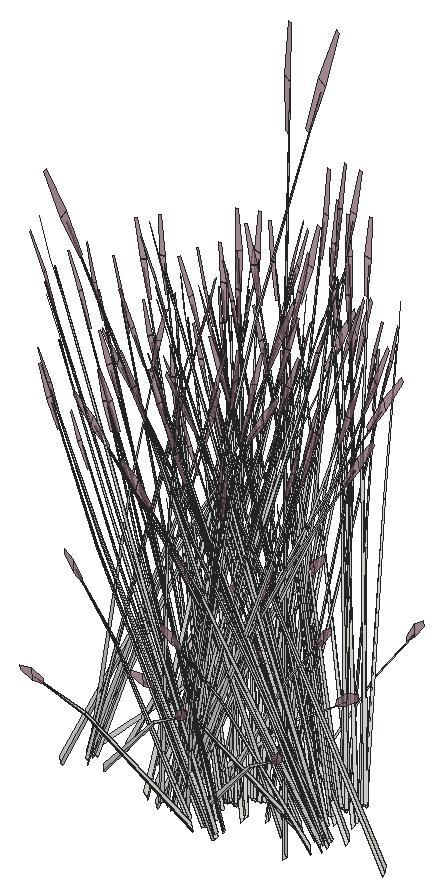
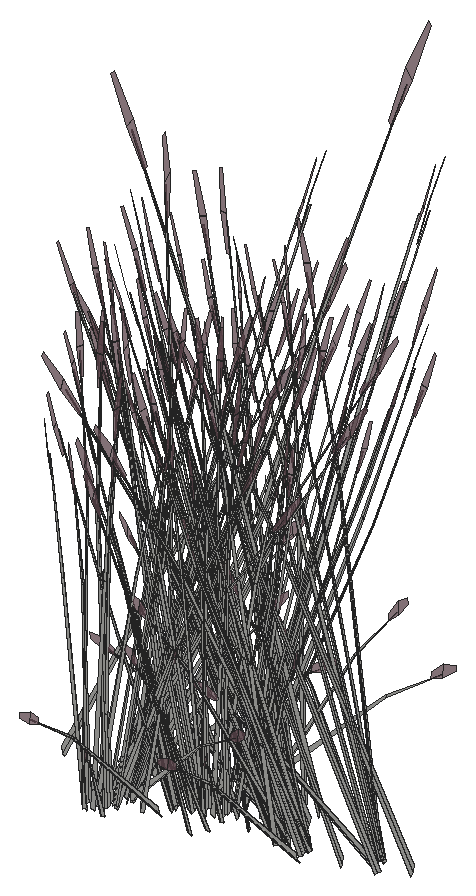
# SketchUp Ruby script. Lengths in inches.
U = 1.inch
M = Sketchup.active_model
def pt(a) = Geom::Point3d.new(a.map { |v| v * U })
def face(e, loops, mat)
  f = e.add_face(loops[0].map { |a| pt(a) })
  loops[1..].each { |l| e.add_face(l.map { |a| pt(a) }).erase! }
  f.material = f.back_material = mat if mat
  f
end
# faces: each face lists its corners as indices into pts; further lists are holes
def faces(e, pts, list, mat = nil) = list.each { |f| face(e, (f[0].is_a?(Array) ? f : [f]).map { |l| l.map { |i| pts[i] } }, mat) }
# xy, xz, yz: faces in a plane at the given z, y or x. An outline is a flat list of corners, or four numbers for a rectangle; further outlines are holes
def ring(l) = l.size == 4 ? [[l[0], l[1]], [l[2], l[1]], [l[2], l[3]], [l[0], l[3]]] : l.each_slice(2).to_a
def flat(e, list, mat, &to3) = list.each { |f| face(e, (f[0].is_a?(Array) ? f : [f]).map { |l| ring(l).map { |u, v| to3.(u, v) } }, mat) }
def xy(e, z, list, mat = nil) = flat(e, list, mat) { |x, y| [x, y, z] }
def xz(e, y, list, mat = nil) = flat(e, list, mat) { |x, z| [x, y, z] }
def yz(e, x, list, mat = nil) = flat(e, list, mat) { |y, z| [x, y, z] }
def lines(e, pts, list) = list.each { |a, b| e.add_line(pt(pts[a]), pt(pts[b])) }
# prism: a flat outline (further loops are holes) pulled along v
def prism(e, loops, v, mat = nil)
  f = face(e, loops, mat); d = Geom::Vector3d.new(v.map { |x| x * U })
  f.pushpull(f.normal.samedirection?(d) ? d.length : -d.length)
end
def box(e, o, s, mat = nil) = prism(e, [[o, [o[0] + s[0], o[1], o[2]], [o[0] + s[0], o[1] + s[1], o[2]], [o[0], o[1] + s[1], o[2]]]], [0, 0, s[2]], mat)
def at(x, y, z, deg = 0) = Geom::Transformation.translation(pt([x, y, z])) * Geom::Transformation.rotation(ORIGIN, Z_AXIS, deg.degrees)
def axes(o, x, y, z) = Geom::Transformation.new([*x, 0, *y, 0, *z, 0, *pt(o).to_a, 1])
def part(name) = M.definitions.add(name)
# library, detail: a bought-in or finely detailed component or shape, given as its bounding box
def library(name, o, s) = part(name).tap { |d| box(d.entities, o, s) }
def detail(e, o, s) = box(e.add_group.entities, o, s)
def put(e, d, t, mat = nil) = e.add_instance(d, t).tap { |i| i.material = mat if mat }
def group(e, t, mat = nil) = e.add_group.tap { |g| g.transformation = t; g.material = mat if mat }.entities
root = M.entities
M.materials.add("LightPink_Translucent").color = [144, 107, 117]
M.materials["LightPink_Translucent"].alpha = 0.75
c1 = part("blade")
p = [[2.15,0.21,22],[0,0.17,0],[0.09,0.45,0],[2.18,0.31,22],[2.29,0.31,22],[0.38,0.45,0],
  [2.48,0.24,33],[2.49,0.24,33],[2.48,0.22,33]]
faces(c1.entities,p,[[0,1,2,3],[4,5,2,3],[6,3,4,7],[8,0,3,6]])
c2 = part("seeds")
p = [[0.3,-0.1,1.38],[-0.01,-0.03,1.59],[-0.01,-0.03,0.03],[0.14,-0.07,-0.07],[0.29,-0.03,3],[0.15,0.01,3.11]]
faces(c2.entities,p,[[0,1,2,3],[1,0,4,5]],"LightPink_Translucent")
c3 = part("blade with seeds")
put(c3.entities,c1,at(0,0,0))
put(c3.entities,c2,axes([2.4,0.25,30.99],[1.5799,-0.05474,1.17369],[-0.12525,1.92788,0.29478],[-0.07173,-0.02425,1.56792]))
put(root,c3,axes([663.24,337.52,268.18],[-0.32734,-0.51701,-0.10093],[0.58097,-0.25407,-0.56021],[0.24483,-0.06821,0.85122]))
put(root,c3,axes([663.46,337.375,267.93],[-0.18381,0.5206,0.39842],[-0.60429,-0.17802,0.32852],[0.23764,-0.03129,0.82444]))
put(root,c3,axes([670.3125,337.49,267.91],[0.08303,0.01531,1.47228],[0.25685,0.50448,-0.13912],[-0.16996,0.13241,0.26054]))
put(root,c3,axes([672.2,336.875,267.89],[-0.17625,0.51936,-0.42412],[-0.60429,-0.17802,-0.32852],[-0.2433,0.04762,0.81151]))
put(root,c3,axes([672.66,335.75,267.89],[-0.47241,0.37822,-0.42412],[-0.41372,-0.39954,-0.32852],[-0.24002,-0.05755,0.81151]))
put(root,c3,axes([666.25,339.77,267.91],[0.08247,0.09194,1.45204],[0.66552,0.03612,-0.22964],[0.06692,0.20277,0.11645]))
put(root,c3,axes([671.99,334.69,267.91],[0.04823,0.05698,1.47228],[-0.23252,0.51221,-0.13912],[-0.23548,0.00371,0.26054]))
put(root,c3,axes([663.08,338.25,267.91],[0.13956,-0.00966,1.45204],[0.38281,-0.44358,-0.22964],[0.24825,0.05855,0.11645]))
put(root,c3,axes([672.53,334.35,267.91],[-0.13998,-0.00403,1.45204],[-0.44565,0.40302,-0.22964],[-0.23779,-0.08235,0.11645]))
put(root,c3,axes([666.59,338.53,268.19],[0.19614,-0.43908,0.29394],[0.57222,0.12807,-0.37948],[0.05247,0.17678,0.72609]))
put(root,c3,axes([663.21,337.08,267.89],[0.17625,-0.51936,-0.42412],[0.60429,0.17802,-0.32852],[0.2433,-0.04762,0.81151]))
put(root,c3,axes([671.96,336.58,267.93],[0.18381,-0.5206,0.39842],[0.60429,0.17802,0.32852],[-0.23764,0.03129,0.82444]))
put(root,c3,axes([672.17,336.43,268.18],[0.32734,0.51701,-0.10093],[-0.58097,0.25407,-0.56021],[-0.24483,0.06821,0.85122]))
put(root,c3,axes([672.91,335.36,268.18],[-0.03484,0.58066,-0.10093],[-0.65957,-0.01587,-0.56021],[-0.25402,-0.04034,0.85122]))
put(root,c3,axes([672.49,335.4,267.76],[-0.37017,-0.35748,-0.29394],[0.42268,-0.3384,0.37948],[-0.21476,-0.05149,0.72609]))
put(root,c3,axes([671.91,336.44,267.93],[-0.23895,-0.38931,0.05337],[0.43573,-0.19055,0.42015],[-0.19208,0.0376,0.64067]))
put(root,c3,axes([673.01,337.52,267.22],[0.1625,-0.17544,1.42242],[0.41029,0.47354,0.11501],[-0.28141,0.21565,0.60807]))
put(root,c3,axes([672.03,337.98,267.76],[-0.56631,0.0816,-0.29394],[-0.14954,-0.46647,0.37948],[-0.16229,0.12529,0.72609]))
put(root,c3,axes([663.58,337.32,267.76],[0.54068,0.15928,-0.29394],[-0.1577,0.46469,0.37948],[0.21769,-0.04261,0.72609]))
put(root,c3,axes([666.71,338.6,268.13],[0.31051,0.46426,-0.58968],[-0.63919,0.25873,0.07116],[0.07261,0.22432,0.83415]))
put(root,c3,axes([662.54,338.32,268.13],[0.65035,0.01375,-0.58968],[-0.04368,0.5789,0.07116],[0.27552,0.06109,0.83415]))
put(root,c3,axes([667.36,340.1,268.6875],[0.44958,-0.32756,-0.05385],[0.41194,0.35875,-0.24415],[0.029,0.10165,0.8053]))
put(root,c3,axes([672.1,337.875,267.93],[-0.16135,-0.52549,0.39842],[0.63294,-0.0912,0.32852],[-0.18654,0.12359,0.82444]))
put(root,c3,axes([664.54,339.06,267.91],[-0.05883,-0.04999,1.47228],[0.12868,-0.53581,-0.13912],[0.23172,-0.03423,0.26054]))
put(root,c3,axes([662.11,336.74,267.22],[-0.26985,0.01293,1.42242],[0.17902,-0.56047,0.11501],[0.38456,0.03467,0.60807]))
put(root,c3,axes([672.43,335.26,268.23],[0.53728,-0.42137,0.44623],[0.46337,0.44748,0.36794],[-0.25207,-0.07773,0.92337]))
put(root,c3,axes([671.98,337.78,267.93],[-0.44663,-0.24013,0.05337],[0.26003,-0.34195,0.42015],[-0.14319,0.11055,0.64067]))
put(root,c3,axes([666.95,338.69,267.89],[0.63954,0.14313,-0.42412],[-0.21921,0.49074,-0.32852],[0.05864,0.19758,0.81151]))
put(root,c3,axes([666.4,338.72,268.18],[0.63664,-0.26583,-0.10093],[0.31286,0.47181,-0.56021],[0.084,0.19882,0.85122]))
put(root,c3,axes([663.1,337.27,268.13],[0.57168,-0.25217,-0.58968],[0.3186,0.51908,0.07116],[0.27622,-0.05897,0.83415]))
put(root,c3,axes([672.89,337.95,267.22],[0.12114,-0.19625,1.42242],[0.50818,0.40613,0.11501],[-0.22925,0.25313,0.60807]))
put(root,c3,axes([672.4,336.59,268.19],[0.54068,0.15928,0.29394],[-0.1577,0.46469,-0.37948],[-0.21769,0.04261,0.72609]))
put(root,c3,axes([665.02,336.71,267.91],[0.09028,-0.08697,1.45204],[-0.11555,-0.53348,-0.22964],[0.22652,-0.10115,0.11645]))
put(root,c3,axes([672.5,338.03,267.89],[0.16713,0.52135,-0.42412],[-0.63294,0.0912,-0.32852],[-0.18138,0.14003,0.81151]))
put(root,c3,axes([672.68,335.26,267.93],[0.03276,-0.43418,0.05337],[0.49468,0.0119,0.42015],[-0.18949,-0.04543,0.64067]))
put(root,c3,axes([671.51,338.97,267.91],[-0.01617,0.11299,1.45204],[0.45894,0.39307,-0.22964],[-0.12015,0.18588,0.11645]))
put(root,c3,axes([674.2,334.51,268.51],[-0.4342,0.54737,-0.11304],[-0.6288,-0.31535,-0.62743],[-0.21858,-0.15465,0.95337]))
put(root,c3,axes([673.01,335.58,268.19],[0.37017,0.35748,0.29394],[-0.42268,0.3384,-0.37948],[-0.21476,-0.05149,0.72609]))
put(root,c3,axes([673.75,334.97,267.89],[-0.64198,0.13573,-0.42412],[-0.1123,-0.514,-0.32852],[-0.17243,-0.1473,0.81151]))
put(root,c3,axes([672.2,337.66,268.18],[0.60181,0.31483,-0.10093],[-0.34671,0.45593,-0.56021],[-0.17003,0.15849,0.85122]))
put(root,c3,axes([668.18,338.77,267.93],[-0.64708,0.13103,0.39842],[-0.1123,-0.514,0.32852],[0.15218,0.15149,0.82444]))
put(root,c3,axes([668.06,338.875,267.93],[-0.29569,0.36271,0.05337],[-0.42107,-0.21117,0.42015],[0.13613,0.11629,0.64067]))
put(root,c3,axes([667.31,337.68,267.22],[-0.14872,-0.18332,1.42242],[0.6872,-0.15433,0.11501],[0.15531,0.28779,0.60807]))
put(root,c3,axes([676.87,339.23,267.22],[0.26985,-0.01293,1.42242],[-0.17902,0.56047,0.11501],[-0.38456,-0.03467,0.60807]))
put(root,c3,axes([671.21,339.03,268.6875],[0.5741,0.15241,-0.05385],[-0.1766,0.46909,-0.24415],[-0.0939,0.07122,0.8053]))
put(root,c3,axes([672.49,337.7,268.19],[0.56631,-0.0816,0.29394],[0.14954,0.46647,-0.37948],[-0.16229,0.12529,0.72609]))
put(root,c3,axes([667.96,338.46,268.19],[-0.10048,-0.4599,0.29394],[0.5744,-0.12144,-0.37948],[0.15428,0.13179,0.72609]))
put(root,c3,axes([673.03,338.94,267.93],[-0.46327,-0.38957,0.39842],[0.49199,-0.33598,0.32852],[-0.08546,0.18277,0.82444]))
put(root,c3,axes([676.98,340.21,267.22],[0.22574,-0.12077,1.42242],[0.19004,0.55807,0.11501],[-0.35439,0.12613,0.60807]))
put(root,c3,axes([668.35,335.8125,267.71],[-0.56218,-0.29666,1.14775],[0.59361,-0.46189,0.49522],[0.18138,0.27836,1.10941]))
put(root,c3,axes([667.4,339.1,267.91],[0.00193,-0.06913,1.47228],[0.55753,-0.30498,-0.13912],[0.19366,0.10886,0.26054]))
put(root,c3,axes([672.86,338.9,267.93],[-0.53464,-0.0266,0.05337],[0.01466,-0.40172,0.42015],[-0.05594,0.15388,0.64067]))
put(root,c3,axes([673.03,339.06,267.76],[-0.4402,0.30062,-0.29394],[-0.41671,-0.34326,0.37948],[-0.0634,0.1744,0.72609]))
put(root,c3,axes([678.28,339.63,266.77],[0.18493,-0.0826,1.46963],[0.06377,0.5767,0.11501],[-0.40056,0.07652,0.52526]))
put(root,c3,axes([674.16,334.96,268.19],[0.10048,0.4599,0.29394],[-0.5744,0.12144,-0.37948],[-0.15428,-0.13179,0.72609]))
put(root,c3,axes([671.46,340.125,267.91],[0.07381,-0.03447,1.47228],[0.61004,0.22929,-0.13912],[-0.01434,0.19091,0.26054]))
put(root,c3,axes([675.34,338.07,266.76],[0.56221,0.23024,1.25546],[-0.55078,0.49601,0.49647],[-0.2467,-0.29398,1.05249]))
put(root,c3,axes([669.63,335.72,268.19],[-0.56631,0.0816,0.29394],[-0.14954,-0.46647,-0.37948],[0.16229,-0.12529,0.72609]))
put(root,c3,axes([676.29,340.02,267.91],[-0.10624,0.07413,1.45204],[0.00904,0.54162,-0.22964],[-0.24352,0.07044,0.11645]))
put(root,c3,axes([677.68,338.71,268.13],[-0.65035,-0.01375,-0.58968],[0.04368,-0.5789,0.07116],[-0.27552,-0.06109,0.83415]))
put(root,c3,axes([673.32,338.74,268.43],[-0.01693,0.52814,-0.65454],[-0.71285,-0.03547,0.07899],[-0.07523,0.22375,0.92591]))
put(root,c3,axes([676.63,339.71,267.76],[-0.54068,-0.15928,-0.29394],[0.1577,-0.46469,0.37948],[-0.21769,0.04261,0.72609]))
put(root,c3,axes([677.38,338.33,267.22],[0.24166,0.09837,1.42242],[-0.50011,0.41269,0.11501],[-0.3117,-0.18617,0.60807]))
put(root,c3,axes([667.91,338.7,268.18],[0.38768,-0.48872,-0.10093],[0.56143,0.28156,-0.56021],[0.19516,0.13808,0.85122]))
put(root,c3,axes([675.11,340.5625,267.91],[0.08303,0.01531,1.47228],[0.25685,0.50448,-0.13912],[-0.16996,0.13241,0.26054]))
put(root,c3,axes([677,339.94,267.89],[-0.17625,0.51936,-0.42412],[-0.60429,-0.17802,-0.32852],[-0.2433,0.04762,0.81151]))
put(root,c3,axes([673.08,339.48,266.79],[0.01429,-0.29475,1.28107],[0.64291,0.15569,0.17703],[-0.0557,0.31414,0.60492]))
put(root,c3,axes([677.46,338.82,267.89],[-0.47241,0.37822,-0.42412],[-0.41372,-0.39954,-0.32852],[-0.24002,-0.05755,0.81151]))
put(root,c3,axes([668.37,338.45,267.89],[0.64198,-0.13573,-0.42412],[0.1123,0.514,-0.32852],[0.17243,0.1473,0.81151]))
put(root,c3,axes([669.11,337.84,268.19],[-0.37017,-0.35748,0.29394],[0.42268,-0.3384,-0.37948],[0.21476,0.05149,0.72609]))
put(root,c3,axes([676.8,337.76,267.91],[0.04823,0.05698,1.47228],[-0.23252,0.51221,-0.13912],[-0.23548,0.00371,0.26054]))
put(root,c3,axes([669.44,338.16,267.93],[-0.03276,0.43418,0.05337],[-0.49468,-0.0119,0.42015],[0.18949,0.04543,0.64067]))
put(root,c3,axes([677.33,337.42,267.91],[-0.13998,-0.00403,1.45204],[-0.44565,0.40302,-0.22964],[-0.23779,-0.08235,0.11645]))
put(root,c3,axes([673.46,338.91,268.15],[0.46573,0.38364,-0.47077],[-0.49199,0.33598,-0.36465],[-0.07086,0.19492,0.90078]))
put(root,c3,axes([669.49,338.02,267.93],[-0.47971,0.37622,0.39842],[-0.41372,-0.39954,0.32852],[0.22506,0.0694,0.82444]))
put(root,c3,axes([673.26,338.63,268.19],[0.4402,-0.30062,0.29394],[0.41671,0.34326,-0.37948],[-0.0634,0.1744,0.72609]))
put(root,c3,axes([676.76,339.65,267.93],[0.18381,-0.5206,0.39842],[0.60429,0.17802,0.32852],[-0.23764,0.03129,0.82444]))
put(root,c3,axes([676.98,339.5,268.18],[0.32734,0.51701,-0.10093],[-0.58097,0.25407,-0.56021],[-0.24483,0.06821,0.85122]))
put(root,c3,axes([676.21,336.97,266.36],[-0.01777,-0.53759,1.17256],[0.80434,0.13935,0.49647],[-0.19024,0.29416,1.1068]))
put(root,c3,axes([670.74,338.08,267.26],[-0.12452,-0.47997,-0.02898],[0.58854,-0.11034,-0.1314],[0.1229,0.03043,0.43341]))
put(root,c3,axes([669.72,336.83,268.19],[-0.54068,-0.15928,0.29394],[0.1577,-0.46469,-0.37948],[0.21769,-0.04261,0.72609]))
put(root,c3,axes([677.71,338.43,268.18],[-0.03484,0.58066,-0.10093],[-0.65957,-0.01587,-0.56021],[-0.25402,-0.04034,0.85122]))
put(root,c3,axes([677.29,338.47,267.76],[-0.37017,-0.35748,-0.29394],[0.42268,-0.3384,0.37948],[-0.21476,-0.05149,0.72609]))
put(root,c3,axes([676.71,339.51,267.93],[-0.23895,-0.38931,0.05337],[0.43573,-0.19055,0.42015],[-0.19208,0.0376,0.64067]))
put(root,c3,axes([677.81,340.59,267.22],[0.1625,-0.17544,1.42242],[0.41029,0.47354,0.11501],[-0.28141,0.21565,0.60807]))
put(root,c3,axes([676.83,341.05,267.76],[-0.56631,0.0816,-0.29394],[-0.14954,-0.46647,0.37948],[-0.16229,0.12529,0.72609]))
put(root,c3,axes([672.98,338.71,268.48],[0.71502,0.02829,-0.11203],[-0.01954,0.53563,-0.62183],[-0.04967,0.20629,0.94486]))
put(root,c3,axes([670.14,335.64,267.93],[0.44663,0.24013,0.05337],[-0.26003,0.34195,0.42015],[0.14319,-0.11055,0.64067]))
put(root,c3,axes([673.99,338.36,267.22],[-0.01592,-0.21915,1.42242],[0.69015,0.14538,0.11501],[-0.04269,0.3123,0.60807]))
put(root,c3,axes([676.9,340.95,267.93],[-0.16135,-0.52549,0.39842],[0.63294,-0.0912,0.32852],[-0.18654,0.12359,0.82444]))
put(root,c3,axes([670.02,335.54,267.93],[0.16135,0.52549,0.39842],[-0.63294,0.0912,0.32852],[0.18654,-0.12359,0.82444]))
put(root,c3,axes([677.23,338.33,268.23],[0.53728,-0.42137,0.44623],[0.46337,0.44748,0.36794],[-0.25207,-0.07773,0.92337]))
put(root,c3,axes([676.78,340.85,267.93],[-0.44663,-0.24013,0.05337],[0.26003,-0.34195,0.42015],[-0.14319,0.11055,0.64067]))
put(root,c3,axes([668.3,337.11,267.22],[-0.24166,-0.09837,1.42242],[0.50011,-0.41269,0.11501],[0.3117,0.18617,0.60807]))
put(root,c3,axes([671.4,335.625,267.91],[-0.08498,-0.00434,1.47228],[-0.35287,-0.46464,-0.13912],[0.14171,-0.15278,0.26054]))
put(root,c3,axes([677.6875,341.02,267.22],[0.12114,-0.19625,1.42242],[0.50818,0.40613,0.11501],[-0.22925,0.25313,0.60807]))
put(root,c3,axes([670.09,335.44,267.76],[0.56631,-0.0816,-0.29394],[0.14954,0.46647,0.37948],[0.16229,-0.12529,0.72609]))
put(root,c3,axes([670.21,336.98,267.93],[0.23895,0.38931,0.05337],[-0.43573,0.19055,0.42015],[0.19208,-0.0376,0.64067]))
put(root,c3,axes([669.63,338.02,267.76],[0.37017,0.35748,-0.29394],[-0.42268,0.3384,0.37948],[0.21476,0.05149,0.72609]))
put(root,c3,axes([669.21,338.0625,268.18],[0.03484,-0.58066,-0.10093],[0.65957,0.01587,-0.56021],[0.25402,0.04034,0.85122]))
put(root,c3,axes([677.2,339.66,268.19],[0.54068,0.15928,0.29394],[-0.1577,0.46469,-0.37948],[-0.21769,0.04261,0.72609]))
put(root,c3,axes([669.95,336.99,268.18],[-0.32734,-0.51701,-0.10093],[0.58097,-0.25407,-0.56021],[0.24483,-0.06821,0.85122]))
put(root,c3,axes([670.16,336.84,267.93],[-0.18381,0.5206,0.39842],[-0.60429,-0.17802,0.32852],[0.23764,-0.03129,0.82444]))
put(root,c3,axes([677.3,341.1,267.89],[0.16713,0.52135,-0.42412],[-0.63294,0.0912,-0.32852],[-0.18138,0.14003,0.81151]))
put(root,c3,axes([677.48,338.33,267.93],[0.03276,-0.43418,0.05337],[0.49468,0.0119,0.42015],[-0.18949,-0.04543,0.64067]))
put(root,c3,axes([676.31,342.04,267.91],[-0.01617,0.11299,1.45204],[0.45894,0.39307,-0.22964],[-0.12015,0.18588,0.11645]))
put(root,c3,axes([679,337.58,268.51],[-0.4342,0.54737,-0.11304],[-0.6288,-0.31535,-0.62743],[-0.21858,-0.15465,0.95337]))
put(root,c3,axes([674.48,339.49,268.2],[-0.64106,-0.14927,0.44225],[0.21921,-0.49074,0.36465],[0.03852,0.19299,0.91512]))
put(root,c3,axes([677.8125,338.65,268.19],[0.37017,0.35748,0.29394],[-0.42268,0.3384,-0.37948],[-0.21476,-0.05149,0.72609]))
put(root,c3,axes([674.3125,339.52,267.93],[-0.47939,0.19405,0.05337],[-0.23464,-0.35385,0.42015],[0.0463,0.15598,0.64067]))
put(root,c3,axes([678.81,338.02,268.13],[-0.55475,-0.27598,-0.58968],[0.39425,-0.48361,0.07116],[-0.20099,-0.16478,0.83415]))
put(root,c3,axes([678.55,338.04,267.89],[-0.64198,0.13573,-0.42412],[-0.1123,-0.514,-0.32852],[-0.17243,-0.1473,0.81151]))
put(root,c3,axes([669.78,337.72,267.91],[0.13956,-0.00966,1.45204],[0.38281,-0.44358,-0.22964],[0.24825,0.05855,0.11645]))
put(root,c3,axes([669.92,336.55,267.89],[0.17625,-0.51936,-0.42412],[0.60429,0.17802,-0.32852],[0.2433,-0.04762,0.81151]))
put(root,c3,axes([677,340.73,268.18],[0.60181,0.31483,-0.10093],[-0.34671,0.45593,-0.56021],[-0.17003,0.15849,0.85122]))
put(root,c3,axes([670.29,336.78,267.76],[0.54068,0.15928,-0.29394],[-0.1577,0.46469,0.37948],[0.21769,-0.04261,0.72609]))
put(root,c3,axes([676.01,342.1,268.6875],[0.5741,0.15241,-0.05385],[-0.1766,0.46909,-0.24415],[-0.0939,0.07122,0.8053]))
put(root,c3,axes([674.55,339.59,267.76],[-0.19614,0.43908,-0.29394],[-0.57222,-0.12807,0.37948],[0.05247,0.17678,0.72609]))
put(root,c3,axes([669.24,337.78,268.13],[0.65035,0.01375,-0.58968],[-0.04368,0.5789,0.07116],[0.27552,0.06109,0.83415]))
put(root,c3,axes([677.29,340.77,268.19],[0.56631,-0.0816,0.29394],[0.14954,0.46647,-0.37948],[-0.16229,0.12529,0.72609]))
put(root,c3,axes([671.25,338.53,267.91],[-0.05883,-0.04999,1.47228],[0.12868,-0.53581,-0.13912],[0.23172,-0.03423,0.26054]))
put(root,c3,axes([668.8125,336.21,267.22],[-0.26985,0.01293,1.42242],[0.17902,-0.56047,0.11501],[0.38456,0.03467,0.60807]))
put(root,c3,axes([678.83,336.28,267.91],[-0.01214,0.06844,1.47228],[-0.59861,0.24837,-0.13912],[-0.17615,-0.12696,0.26054]))
put(root,c3,axes([674.15,340.37,267.91],[0.08247,0.09194,1.45204],[0.66552,0.03612,-0.22964],[0.06692,0.20277,0.11645]))
put(root,c3,axes([678.375,337.75,267.22],[0.14872,0.18332,1.42242],[-0.6872,0.15433,0.11501],[-0.15531,-0.28779,0.60807]))
put(root,c3,axes([682.3,337.68,267.22],[0.26985,-0.01293,1.42242],[-0.17902,0.56047,0.11501],[-0.38456,-0.03467,0.60807]))
put(root,c3,axes([669.8,336.73,268.13],[0.57168,-0.25217,-0.58968],[0.3186,0.51908,0.07116],[0.27622,-0.05897,0.83415]))
put(root,c3,axes([677.83,342.01,267.93],[-0.46327,-0.38957,0.39842],[0.49199,-0.33598,0.32852],[-0.08546,0.18277,0.82444]))
put(root,c3,axes([678.62,337.66,267.76],[-0.10048,-0.4599,-0.29394],[0.5744,-0.12144,0.37948],[-0.15428,-0.13179,0.72609]))
put(root,c3,axes([674.49,339.125,268.19],[0.19614,-0.43908,0.29394],[0.57222,0.12807,-0.37948],[0.05247,0.17678,0.72609]))
put(root,c3,axes([677.66,341.97,267.93],[-0.53464,-0.0266,0.05337],[0.01466,-0.40172,0.42015],[-0.05594,0.15388,0.64067]))
put(root,c3,axes([671.72,336.18,267.91],[0.09028,-0.08697,1.45204],[-0.11555,-0.53348,-0.22964],[0.22652,-0.10115,0.11645]))
put(root,c3,axes([677.83,342.13,267.76],[-0.4402,0.30062,-0.29394],[-0.41671,-0.34326,0.37948],[-0.0634,0.1744,0.72609]))
